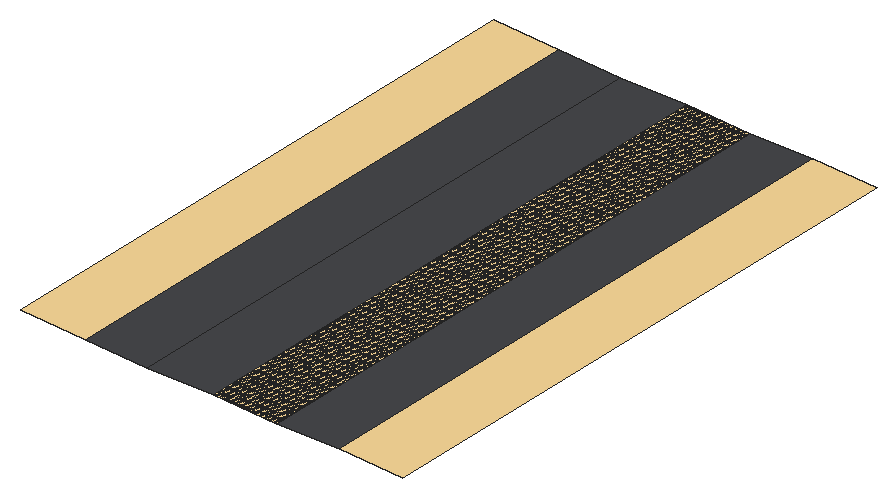
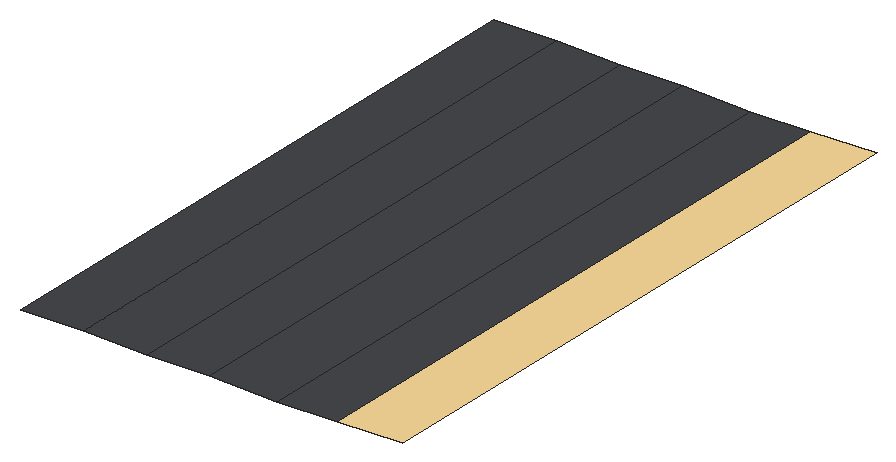
# SketchUp Ruby script. Lengths in inches.
U = 1.inch
M = Sketchup.active_model
def pt(a) = Geom::Point3d.new(a.map { |v| v * U })
def face(e, loops, mat)
  f = e.add_face(loops[0].map { |a| pt(a) })
  loops[1..].each { |l| e.add_face(l.map { |a| pt(a) }).erase! }
  f.material = f.back_material = mat if mat
  f
end
# faces: each face lists its corners as indices into pts; further lists are holes
def faces(e, pts, list, mat = nil) = list.each { |f| face(e, (f[0].is_a?(Array) ? f : [f]).map { |l| l.map { |i| pts[i] } }, mat) }
# xy, xz, yz: faces in a plane at the given z, y or x. An outline is a flat list of corners, or four numbers for a rectangle; further outlines are holes
def ring(l) = l.size == 4 ? [[l[0], l[1]], [l[2], l[1]], [l[2], l[3]], [l[0], l[3]]] : l.each_slice(2).to_a
def flat(e, list, mat, &to3) = list.each { |f| face(e, (f[0].is_a?(Array) ? f : [f]).map { |l| ring(l).map { |u, v| to3.(u, v) } }, mat) }
def xy(e, z, list, mat = nil) = flat(e, list, mat) { |x, y| [x, y, z] }
def xz(e, y, list, mat = nil) = flat(e, list, mat) { |x, z| [x, y, z] }
def yz(e, x, list, mat = nil) = flat(e, list, mat) { |y, z| [x, y, z] }
def lines(e, pts, list) = list.each { |a, b| e.add_line(pt(pts[a]), pt(pts[b])) }
# prism: a flat outline (further loops are holes) pulled along v
def prism(e, loops, v, mat = nil)
  f = face(e, loops, mat); d = Geom::Vector3d.new(v.map { |x| x * U })
  f.pushpull(f.normal.samedirection?(d) ? d.length : -d.length)
end
def box(e, o, s, mat = nil) = prism(e, [[o, [o[0] + s[0], o[1], o[2]], [o[0] + s[0], o[1] + s[1], o[2]], [o[0], o[1] + s[1], o[2]]]], [0, 0, s[2]], mat)
def at(x, y, z, deg = 0) = Geom::Transformation.translation(pt([x, y, z])) * Geom::Transformation.rotation(ORIGIN, Z_AXIS, deg.degrees)
def axes(o, x, y, z) = Geom::Transformation.new([*x, 0, *y, 0, *z, 0, *pt(o).to_a, 1])
def part(name) = M.definitions.add(name)
# library, detail: a bought-in or finely detailed component or shape, given as its bounding box
def library(name, o, s) = part(name).tap { |d| box(d.entities, o, s) }
def detail(e, o, s) = box(e.add_group.entities, o, s)
def put(e, d, t, mat = nil) = e.add_instance(d, t).tap { |i| i.material = mat if mat }
def group(e, t, mat = nil) = e.add_group.tap { |g| g.transformation = t; g.material = mat if mat }.entities
root = M.entities
M.materials.add("1432 AP 8245 TAR ROAD").color = [71, 72, 75]
M.materials.add("Outer Light").color = [251, 217, 152]
xy(root,171.3,[[278.36,95.37,278.52,96.87]],"1432 AP 8245 TAR ROAD")
xy(root,171.3,[[278.36,95.37,278.52,96.87]],"Outer Light")
xy(root,171.31,[[278.03,95.37,278.2,96.87]],"1432 AP 8245 TAR ROAD")
xy(root,171.31,[[278.03,95.37,278.2,96.87]],"Outer Light")
p = [[277.71,96.87,171.33],[277.875,96.87,171.32],[277.875,95.37,171.32],[277.71,95.37,171.33],[278.03,96.87,171.31],[278.03,95.37,171.31],
  [277.875,95.37,171.32],[278.03,95.37,171.31],[278.03,96.87,171.31],[277.875,96.87,171.32],[278.2,96.87,171.31],[278.36,96.87,171.3],
  [278.36,95.37,171.3],[278.2,95.37,171.31],[278.2,95.37,171.31],[278.36,95.37,171.3],[278.36,96.87,171.3],[278.2,96.87,171.31],
  [278.52,96.87,171.3],[278.68,96.87,171.29],[278.68,95.37,171.29],[278.52,95.37,171.3],[278.52,95.37,171.3],[278.68,95.37,171.29],
  [278.68,96.87,171.29],[278.52,96.87,171.3]]
faces(root,p,[[0,1,2,3],[1,4,5,2],[10,11,12,13],[18,19,20,21]],"Outer Light")
faces(root,p,[[6,7,8,9],[14,15,16,17],[22,23,24,25]],"1432 AP 8245 TAR ROAD")
